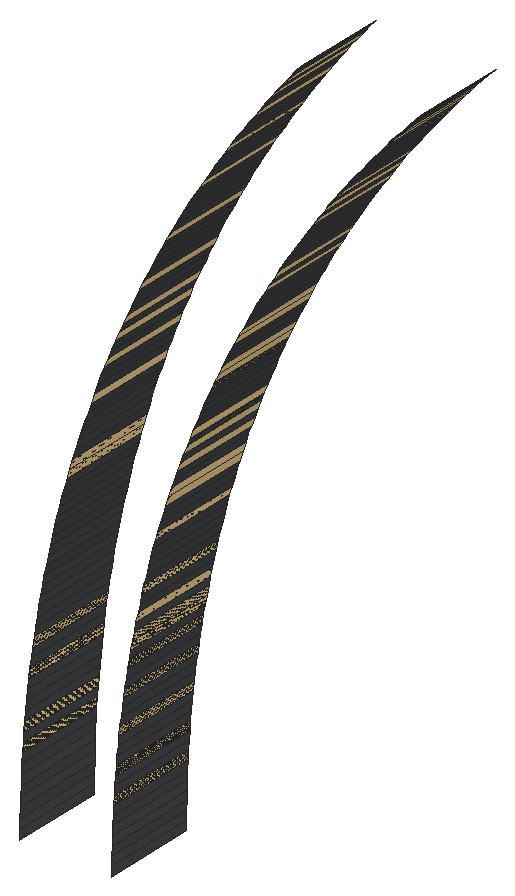
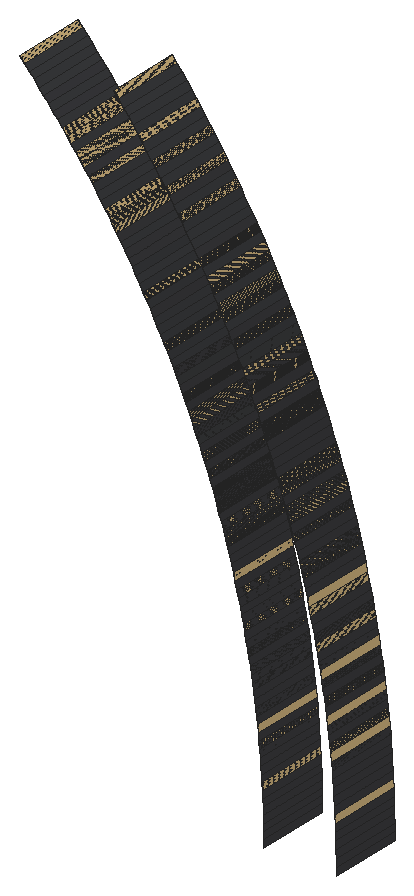
# SketchUp Ruby script. Lengths in inches.
U = 1.inch
M = Sketchup.active_model
def pt(a) = Geom::Point3d.new(a.map { |v| v * U })
def face(e, loops, mat)
  f = e.add_face(loops[0].map { |a| pt(a) })
  loops[1..].each { |l| e.add_face(l.map { |a| pt(a) }).erase! }
  f.material = f.back_material = mat if mat
  f
end
# faces: each face lists its corners as indices into pts; further lists are holes
def faces(e, pts, list, mat = nil) = list.each { |f| face(e, (f[0].is_a?(Array) ? f : [f]).map { |l| l.map { |i| pts[i] } }, mat) }
# xy, xz, yz: faces in a plane at the given z, y or x. An outline is a flat list of corners, or four numbers for a rectangle; further outlines are holes
def ring(l) = l.size == 4 ? [[l[0], l[1]], [l[2], l[1]], [l[2], l[3]], [l[0], l[3]]] : l.each_slice(2).to_a
def flat(e, list, mat, &to3) = list.each { |f| face(e, (f[0].is_a?(Array) ? f : [f]).map { |l| ring(l).map { |u, v| to3.(u, v) } }, mat) }
def xy(e, z, list, mat = nil) = flat(e, list, mat) { |x, y| [x, y, z] }
def xz(e, y, list, mat = nil) = flat(e, list, mat) { |x, z| [x, y, z] }
def yz(e, x, list, mat = nil) = flat(e, list, mat) { |y, z| [x, y, z] }
def lines(e, pts, list) = list.each { |a, b| e.add_line(pt(pts[a]), pt(pts[b])) }
# prism: a flat outline (further loops are holes) pulled along v
def prism(e, loops, v, mat = nil)
  f = face(e, loops, mat); d = Geom::Vector3d.new(v.map { |x| x * U })
  f.pushpull(f.normal.samedirection?(d) ? d.length : -d.length)
end
def box(e, o, s, mat = nil) = prism(e, [[o, [o[0] + s[0], o[1], o[2]], [o[0] + s[0], o[1] + s[1], o[2]], [o[0], o[1] + s[1], o[2]]]], [0, 0, s[2]], mat)
def at(x, y, z, deg = 0) = Geom::Transformation.translation(pt([x, y, z])) * Geom::Transformation.rotation(ORIGIN, Z_AXIS, deg.degrees)
def axes(o, x, y, z) = Geom::Transformation.new([*x, 0, *y, 0, *z, 0, *pt(o).to_a, 1])
def part(name) = M.definitions.add(name)
# library, detail: a bought-in or finely detailed component or shape, given as its bounding box
def library(name, o, s) = part(name).tap { |d| box(d.entities, o, s) }
def detail(e, o, s) = box(e.add_group.entities, o, s)
def put(e, d, t, mat = nil) = e.add_instance(d, t).tap { |i| i.material = mat if mat }
def group(e, t, mat = nil) = e.add_group.tap { |g| g.transformation = t; g.material = mat if mat }.entities
root = M.entities
M.materials.add("1432 AP 8245 TAR ROAD").color = [71, 72, 75]
M.materials.add("Outer Light").color = [251, 217, 152]
yz(root,258.5,[[95.37,560.79,96.87,560.95],[95.37,560.95,96.87,561.11]],"1432 AP 8245 TAR ROAD")
yz(root,258.5,[[95.37,560.79,96.87,560.95],[95.37,560.95,96.87,561.11]],"Outer Light")
yz(root,258.51,[[95.37,561.28,96.87,561.4375]],"1432 AP 8245 TAR ROAD")
yz(root,258.51,[[95.37,561.28,96.87,561.4375]],"Outer Light")
yz(root,258.52,[[95.37,561.6,96.87,561.76]],"1432 AP 8245 TAR ROAD")
yz(root,258.52,[[95.37,561.6,96.87,561.76]],"Outer Light")
yz(root,260,[[95.37,560.79,96.87,560.94],[95.37,560.94,96.87,561.09]],"1432 AP 8245 TAR ROAD")
yz(root,260,[[95.37,560.79,96.87,560.94],[95.37,560.94,96.87,561.09]],"Outer Light")
yz(root,260.01,[[95.37,561.24,96.87,561.39],[95.37,561.39,96.87,561.54]],"1432 AP 8245 TAR ROAD")
yz(root,260.01,[[95.37,561.24,96.87,561.39],[95.37,561.39,96.87,561.54]],"Outer Light")
p = [[258.51,95.37,561.28],[258.5,95.37,561.11],[258.5,96.87,561.11],[258.51,96.87,561.28],[258.51,96.87,561.28],[258.5,96.87,561.11],
  [258.5,95.37,561.11],[258.51,95.37,561.28],[260,95.37,561.09],[260.01,95.37,561.24],[260.01,96.87,561.24],[260,96.87,561.09],
  [260,96.87,561.09],[260.01,96.87,561.24],[260.01,95.37,561.24],[260,95.37,561.09],[258.52,95.37,561.6],[258.51,95.37,561.4375],
  [258.51,96.87,561.4375],[258.52,96.87,561.6],[258.52,96.87,561.6],[258.51,96.87,561.4375],[258.51,95.37,561.4375],[258.52,95.37,561.6],
  [260.01,95.37,561.54],[260.02,95.37,561.6875],[260.02,96.87,561.6875],[260.01,96.87,561.54],[260.01,96.87,561.54],[260.02,96.87,561.6875],
  [260.02,95.37,561.6875],[260.01,95.37,561.54],[260.03,95.37,561.84],[260.03,96.87,561.84],[260.03,96.87,561.84],[260.03,95.37,561.84],
  [258.53,95.37,561.92],[258.52,95.37,561.76],[258.52,96.87,561.76],[258.53,96.87,561.92],[258.53,96.87,561.92],[258.52,96.87,561.76],
  [258.52,95.37,561.76],[258.53,95.37,561.92],[260.04,95.37,561.99],[260.04,96.87,561.99],[260.04,96.87,561.99],[260.04,95.37,561.99],
  [258.54,95.37,562.08],[258.54,96.87,562.08],[258.54,96.87,562.08],[258.54,95.37,562.08],[260.05,95.37,562.13],[260.05,96.87,562.13],
  [260.05,96.87,562.13],[260.05,95.37,562.13],[258.55,95.37,562.24],[258.55,96.87,562.24],[258.55,96.87,562.24],[258.55,95.37,562.24],
  [260.06,95.37,562.28],[260.06,96.87,562.28],[260.06,96.87,562.28],[260.06,95.37,562.28],[258.5625,95.37,562.4],[258.5625,96.87,562.4],
  [258.5625,96.87,562.4],[258.5625,95.37,562.4],[260.07,95.37,562.43],[260.07,96.87,562.43],[260.07,96.87,562.43],[260.07,95.37,562.43],
  [258.58,95.37,562.5625],[258.58,96.87,562.5625],[258.58,96.87,562.5625],[258.58,95.37,562.5625],[260.08,95.37,562.58],[260.08,96.87,562.58],
  [260.08,96.87,562.58],[260.08,95.37,562.58],[258.59,95.37,562.72],[258.59,96.87,562.72],[258.59,96.87,562.72],[258.59,95.37,562.72],
  [260.1,95.37,562.73],[260.1,96.87,562.73],[260.1,96.87,562.73],[260.1,95.37,562.73],[258.61,95.37,562.88],[258.61,96.87,562.88],
  [258.61,96.87,562.88],[258.61,95.37,562.88],[260.11,95.37,562.88],[260.11,96.87,562.88],[260.11,96.87,562.88],[260.11,95.37,562.88],
  [258.625,95.37,563.04],[258.625,96.87,563.04],[258.625,96.87,563.04],[258.625,95.37,563.04],[260.13,95.37,563.03],[260.13,96.87,563.03],
  [260.13,96.87,563.03],[260.13,95.37,563.03],[258.64,95.37,563.2],[258.64,96.87,563.2],[258.64,96.87,563.2],[258.64,95.37,563.2],
  [260.15,95.37,563.17],[260.15,96.87,563.17],[260.15,96.87,563.17],[260.15,95.37,563.17],[258.66,95.37,563.36],[258.66,96.87,563.36],
  [258.66,96.87,563.36],[258.66,95.37,563.36],[260.17,95.37,563.32],[260.17,96.87,563.32],[260.17,96.87,563.32],[260.17,95.37,563.32],
  [260.19,95.37,563.47],[260.19,96.87,563.47],[260.19,96.87,563.47],[260.19,95.37,563.47],[258.68,95.37,563.52],[258.68,96.87,563.52],
  [258.68,96.87,563.52],[258.68,95.37,563.52],[258.7,95.37,563.68],[258.7,96.87,563.68],[258.7,96.87,563.68],[258.7,95.37,563.68],
  [260.21,95.37,563.62],[260.21,96.87,563.62],[260.21,96.87,563.62],[260.21,95.37,563.62],[260.23,95.37,563.76],[260.23,96.87,563.76],
  [260.23,96.87,563.76],[260.23,95.37,563.76],[258.73,95.37,563.84],[258.73,96.87,563.84],[258.73,96.87,563.84],[258.73,95.37,563.84],
  [258.75,95.37,564],[258.75,96.87,564],[258.75,96.87,564],[258.75,95.37,564],[260.26,95.37,563.91],[260.26,96.87,563.91],
  [260.26,96.87,563.91],[260.26,95.37,563.91],[260.28,95.37,564.06],[260.28,96.87,564.06],[260.28,96.87,564.06],[260.28,95.37,564.06],
  [258.78,95.37,564.16],[258.78,96.87,564.16],[258.78,96.87,564.16],[258.78,95.37,564.16],[260.31,95.37,564.21],[260.31,96.87,564.21],
  [260.31,96.87,564.21],[260.31,95.37,564.21],[258.81,95.37,564.32],[258.81,96.87,564.32],[258.81,96.87,564.32],[258.81,95.37,564.32],
  [260.34,95.37,564.35],[260.34,96.87,564.35],[260.34,96.87,564.35],[260.34,95.37,564.35],[258.83,95.37,564.48],[258.83,96.87,564.48],
  [258.83,96.87,564.48],[258.83,95.37,564.48],[260.37,95.37,564.5],[260.37,96.87,564.5],[260.37,96.87,564.5],[260.37,95.37,564.5],
  [258.86,95.37,564.63],[258.86,96.87,564.63],[258.86,96.87,564.63],[258.86,95.37,564.63],[260.39,95.37,564.65],[260.39,96.87,564.65],
  [260.39,96.87,564.65],[260.39,95.37,564.65],[258.89,95.37,564.79],[258.89,96.87,564.79],[258.89,96.87,564.79],[258.89,95.37,564.79],
  [260.43,95.37,564.79],[260.43,96.87,564.79],[260.43,96.87,564.79],[260.43,95.37,564.79],[258.93,95.37,564.95],[258.93,96.87,564.95],
  [258.93,96.87,564.95],[258.93,95.37,564.95],[260.46,95.37,564.9375],[260.46,96.87,564.9375],[260.46,96.87,564.9375],[260.46,95.37,564.9375],
  [258.96,95.37,565.11],[258.96,96.87,565.11],[258.96,96.87,565.11],[258.96,95.37,565.11],[260.49,95.37,565.08],[260.49,96.87,565.08],
  [260.49,96.87,565.08],[260.49,95.37,565.08],[258.99,95.37,565.26],[258.99,96.87,565.26],[258.99,96.87,565.26],[258.99,95.37,565.26],
  [260.52,95.37,565.23],[260.52,96.87,565.23],[260.52,96.87,565.23],[260.52,95.37,565.23],[260.56,95.37,565.37],[260.56,96.87,565.37],
  [260.56,96.87,565.37],[260.56,95.37,565.37],[259.03,95.37,565.42],[259.03,96.87,565.42],[259.03,96.87,565.42],[259.03,95.37,565.42],
  [259.07,95.37,565.58],[259.07,96.87,565.58],[259.07,96.87,565.58],[259.07,95.37,565.58],[260.6,95.37,565.52],[260.6,96.87,565.52],
  [260.6,96.87,565.52],[260.6,95.37,565.52],[260.63,95.37,565.66],[260.63,96.87,565.66],[260.63,96.87,565.66],[260.63,95.37,565.66],
  [259.1,95.37,565.73],[259.1,96.87,565.73],[259.1,96.87,565.73],[259.1,95.37,565.73],[259.14,95.37,565.89],[259.14,96.87,565.89],
  [259.14,96.87,565.89],[259.14,95.37,565.89],[260.67,95.37,565.81],[260.67,96.87,565.81],[260.67,96.87,565.81],[260.67,95.37,565.81],
  [260.71,95.37,565.95],[260.71,96.87,565.95],[260.71,96.87,565.95],[260.71,95.37,565.95],[259.18,95.37,566.05],[259.18,96.87,566.05],
  [259.18,96.87,566.05],[259.18,95.37,566.05],[260.75,95.37,566.09],[260.75,96.87,566.09],[260.75,96.87,566.09],[260.75,95.37,566.09],
  [259.23,95.37,566.2],[259.23,96.87,566.2],[259.23,96.87,566.2],[259.23,95.37,566.2],[260.8,95.37,566.24],[260.8,96.87,566.24],
  [260.8,96.87,566.24],[260.8,95.37,566.24],[259.27,95.37,566.36],[259.27,96.87,566.36],[259.27,96.87,566.36],[259.27,95.37,566.36],
  [260.84,95.37,566.38],[260.84,96.87,566.38],[260.84,96.87,566.38],[260.84,95.37,566.38],[259.3125,95.37,566.51],[259.3125,96.87,566.51],
  [259.3125,96.87,566.51],[259.3125,95.37,566.51],[260.88,95.37,566.52],[260.88,96.87,566.52],[260.88,96.87,566.52],[260.88,95.37,566.52],
  [259.36,95.37,566.67],[259.36,96.87,566.67],[259.36,96.87,566.67],[259.36,95.37,566.67],[260.93,95.37,566.66],[260.93,96.87,566.66],
  [260.93,96.87,566.66],[260.93,95.37,566.66],[259.41,95.37,566.82],[259.41,96.87,566.82],[259.41,96.87,566.82],[259.41,95.37,566.82],
  [260.98,95.37,566.81],[260.98,96.87,566.81],[260.98,96.87,566.81],[260.98,95.37,566.81],[259.45,95.37,566.97],[259.45,96.87,566.97],
  [259.45,96.87,566.97],[259.45,95.37,566.97],[261.02,95.37,566.95],[261.02,96.87,566.95],[261.02,96.87,566.95],[261.02,95.37,566.95],
  [261.07,95.37,567.09],[261.07,96.87,567.09],[261.07,96.87,567.09],[261.07,95.37,567.09],[259.5,95.37,567.125],[259.5,96.87,567.125],
  [259.5,96.87,567.125],[259.5,95.37,567.125],[259.55,95.37,567.28],[259.55,96.87,567.28],[259.55,96.87,567.28],[259.55,95.37,567.28],
  [261.125,95.37,567.23],[261.125,96.87,567.23],[261.125,96.87,567.23],[261.125,95.37,567.23],[261.17,95.37,567.37],[261.17,96.87,567.37],
  [261.17,96.87,567.37],[261.17,95.37,567.37],[259.61,95.37,567.43],[259.61,96.87,567.43],[259.61,96.87,567.43],[259.61,95.37,567.43],
  [259.66,95.37,567.58],[259.66,96.87,567.58],[259.66,96.87,567.58],[259.66,95.37,567.58],[261.23,95.37,567.51],[261.23,96.87,567.51],
  [261.23,96.87,567.51],[261.23,95.37,567.51],[261.28,95.37,567.65],[261.28,96.87,567.65],[261.28,96.87,567.65],[261.28,95.37,567.65],
  [259.71,95.37,567.74],[259.71,96.87,567.74],[259.71,96.87,567.74],[259.71,95.37,567.74],[261.33,95.37,567.79],[261.33,96.87,567.79],
  [261.33,96.87,567.79],[261.33,95.37,567.79],[259.77,95.37,567.89],[259.77,96.87,567.89],[259.77,96.87,567.89],[259.77,95.37,567.89],
  [261.39,95.37,567.92],[261.39,96.87,567.92],[261.39,96.87,567.92],[261.39,95.37,567.92],[259.82,95.37,568.04],[259.82,96.87,568.04],
  [259.82,96.87,568.04],[259.82,95.37,568.04],[261.45,95.37,568.0625],[261.45,96.87,568.0625],[261.45,96.87,568.0625],[261.45,95.37,568.0625],
  [259.88,95.37,568.1875],[259.88,96.87,568.1875],[259.88,96.87,568.1875],[259.88,95.37,568.1875],[261.5,95.37,568.2],[261.5,96.87,568.2],
  [261.5,96.87,568.2],[261.5,95.37,568.2],[259.94,95.37,568.34],[259.94,96.87,568.34],[259.94,96.87,568.34],[259.94,95.37,568.34],
  [261.5625,95.37,568.34],[261.5625,96.87,568.34],[261.5625,96.87,568.34],[261.5625,95.37,568.34],[260,95.37,568.49],[260,96.87,568.49],
  [260,96.87,568.49],[260,95.37,568.49],[261.62,95.37,568.47],[261.62,96.87,568.47],[261.62,96.87,568.47],[261.62,95.37,568.47],
  [260.06,95.37,568.64],[260.06,96.87,568.64],[260.06,96.87,568.64],[260.06,95.37,568.64],[261.68,95.37,568.61],[261.68,96.87,568.61],
  [261.68,96.87,568.61],[261.68,95.37,568.61],[260.12,95.37,568.79],[260.12,96.87,568.79],[260.12,96.87,568.79],[260.12,95.37,568.79],
  [261.75,95.37,568.75],[261.75,96.87,568.75],[261.75,96.87,568.75],[261.75,95.37,568.75],[261.81,95.37,568.88],[261.81,96.87,568.88],
  [261.81,96.87,568.88],[261.81,95.37,568.88],[260.1875,95.37,568.93],[260.1875,96.87,568.93],[260.1875,96.87,568.93],[260.1875,95.37,568.93],
  [260.25,95.37,569.08],[260.25,96.87,569.08],[260.25,96.87,569.08],[260.25,95.37,569.08],[261.87,95.37,569.02],[261.87,96.87,569.02],
  [261.87,96.87,569.02],[261.87,95.37,569.02],[261.9375,95.37,569.15],[261.9375,96.87,569.15],[261.9375,96.87,569.15],[261.9375,95.37,569.15],
  [260.32,95.37,569.23],[260.32,96.87,569.23],[260.32,96.87,569.23],[260.32,95.37,569.23],[260.38,95.37,569.375],[260.38,96.87,569.375],
  [260.38,96.87,569.375],[260.38,95.37,569.375],[262,95.37,569.28],[262,96.87,569.28],[262,96.87,569.28],[262,95.37,569.28],
  [262.07,95.37,569.42],[262.07,96.87,569.42],[262.07,96.87,569.42],[262.07,95.37,569.42],[260.45,95.37,569.52],[260.45,96.87,569.52],
  [260.45,96.87,569.52],[260.45,95.37,569.52],[262.14,95.37,569.55],[262.14,96.87,569.55],[262.14,96.87,569.55],[262.14,95.37,569.55],
  [260.52,95.37,569.67],[260.52,96.87,569.67],[260.52,96.87,569.67],[260.52,95.37,569.67],[262.21,95.37,569.68],[262.21,96.87,569.68],
  [262.21,96.87,569.68],[262.21,95.37,569.68],[260.59,95.37,569.8125],[260.59,96.87,569.8125],[260.59,96.87,569.8125],[260.59,95.37,569.8125],
  [262.28,95.37,569.8125],[262.28,96.87,569.8125],[262.28,96.87,569.8125],[262.28,95.37,569.8125],[260.66,95.37,569.96],[260.66,96.87,569.96],
  [260.66,96.87,569.96],[260.66,95.37,569.96],[262.35,95.37,569.95],[262.35,96.87,569.95],[262.35,96.87,569.95],[262.35,95.37,569.95],
  [262.42,95.37,570.08],[262.42,96.87,570.08],[262.42,96.87,570.08],[262.42,95.37,570.08],[260.73,95.37,570.1],[260.73,96.87,570.1],
  [260.73,96.87,570.1],[260.73,95.37,570.1],[260.81,95.37,570.24],[260.81,96.87,570.24],[260.81,96.87,570.24],[260.81,95.37,570.24],
  [262.5,95.37,570.21],[262.5,96.87,570.21],[262.5,96.87,570.21],[262.5,95.37,570.21],[260.88,95.37,570.38],[260.88,96.87,570.38],
  [260.88,96.87,570.38],[260.88,95.37,570.38],[262.57,95.37,570.34],[262.57,96.87,570.34],[262.57,96.87,570.34],[262.57,95.37,570.34],
  [262.65,95.37,570.46],[262.65,96.87,570.46],[262.65,96.87,570.46],[262.65,95.37,570.46],[260.96,95.37,570.53],[260.96,96.87,570.53],
  [260.96,96.87,570.53],[260.96,95.37,570.53],[261.04,95.37,570.67],[261.04,96.87,570.67],[261.04,96.87,570.67],[261.04,95.37,570.67],
  [262.72,95.37,570.59],[262.72,96.87,570.59],[262.72,96.87,570.59],[262.72,95.37,570.59],[262.8,95.37,570.72],[262.8,96.87,570.72],
  [262.8,96.87,570.72],[262.8,95.37,570.72],[261.11,95.37,570.81],[261.11,96.87,570.81],[261.11,96.87,570.81],[261.11,95.37,570.81],
  [262.88,95.37,570.85],[262.88,96.87,570.85],[262.88,96.87,570.85],[262.88,95.37,570.85],[261.19,95.37,570.95],[261.19,96.87,570.95],
  [261.19,96.87,570.95],[261.19,95.37,570.95],[262.96,95.37,570.97],[262.96,96.87,570.97],[262.96,96.87,570.97],[262.96,95.37,570.97],
  [261.27,95.37,571.09],[261.27,96.87,571.09],[261.27,96.87,571.09],[261.27,95.37,571.09],[263.04,95.37,571.1],[263.04,96.87,571.1],
  [263.04,96.87,571.1],[263.04,95.37,571.1],[261.35,95.37,571.23],[261.35,96.87,571.23],[261.35,96.87,571.23],[261.35,95.37,571.23],
  [263.12,95.37,571.22],[263.12,96.87,571.22],[263.12,96.87,571.22],[263.12,95.37,571.22],[261.4375,95.37,571.37],[261.4375,96.87,571.37],
  [261.4375,96.87,571.37],[261.4375,95.37,571.37],[263.2,95.37,571.35],[263.2,96.87,571.35],[263.2,96.87,571.35],[263.2,95.37,571.35],
  [263.29,95.37,571.47],[263.29,96.87,571.47],[263.29,96.87,571.47],[263.29,95.37,571.47],[261.52,95.37,571.5],[261.52,96.87,571.5],
  [261.52,96.87,571.5],[261.52,95.37,571.5],[261.61,95.37,571.64],[261.61,96.87,571.64],[261.61,96.87,571.64],[261.61,95.37,571.64],
  [263.37,95.37,571.59],[263.37,96.87,571.59],[263.37,96.87,571.59],[263.37,95.37,571.59],[261.69,95.37,571.78],[261.69,96.87,571.78],
  [261.69,96.87,571.78],[261.69,95.37,571.78],[263.46,95.37,571.72],[263.46,96.87,571.72],[263.46,96.87,571.72],[263.46,95.37,571.72],
  [263.54,95.37,571.84],[263.54,96.87,571.84],[263.54,96.87,571.84],[263.54,95.37,571.84],[261.78,95.37,571.91],[261.78,96.87,571.91],
  [261.78,96.87,571.91],[261.78,95.37,571.91],[263.63,95.37,571.96],[263.63,96.87,571.96],[263.63,96.87,571.96],[263.63,95.37,571.96],
  [261.87,95.37,572.05],[261.87,96.87,572.05],[261.87,96.87,572.05],[261.87,95.37,572.05],[261.95,95.37,572.18],[261.95,96.87,572.18],
  [261.95,96.87,572.18],[261.95,95.37,572.18],[263.72,95.37,572.08],[263.72,96.87,572.08],[263.72,96.87,572.08],[263.72,95.37,572.08],
  [263.81,95.37,572.2],[263.81,96.87,572.2],[263.81,96.87,572.2],[263.81,95.37,572.2],[262.04,95.37,572.31],[262.04,96.87,572.31],
  [262.04,96.87,572.31],[262.04,95.37,572.31],[263.9,95.37,572.32],[263.9,96.87,572.32],[263.9,96.87,572.32],[263.9,95.37,572.32],
  [262.14,95.37,572.45],[262.14,96.87,572.45],[262.14,96.87,572.45],[262.14,95.37,572.45],[263.99,95.37,572.4375],[263.99,96.87,572.4375],
  [263.99,96.87,572.4375],[263.99,95.37,572.4375],[262.23,95.37,572.58],[262.23,96.87,572.58],[262.23,96.87,572.58],[262.23,95.37,572.58],
  [264.08,95.37,572.55],[264.08,96.87,572.55],[264.08,96.87,572.55],[264.08,95.37,572.55],[262.32,95.37,572.71],[262.32,96.87,572.71],
  [262.32,96.87,572.71],[262.32,95.37,572.71],[264.17,95.37,572.67],[264.17,96.87,572.67],[264.17,96.87,572.67],[264.17,95.37,572.67],
  [262.42,95.37,572.84],[262.42,96.87,572.84],[262.42,96.87,572.84],[262.42,95.37,572.84],[264.27,95.37,572.79],[264.27,96.87,572.79],
  [264.27,96.87,572.79],[264.27,95.37,572.79],[262.51,95.37,572.97],[262.51,96.87,572.97],[262.51,96.87,572.97],[262.51,95.37,572.97],
  [264.36,95.37,572.9],[264.36,96.87,572.9],[264.36,96.87,572.9],[264.36,95.37,572.9],[264.46,95.37,573.02],[264.46,96.87,573.02],
  [264.46,96.87,573.02],[264.46,95.37,573.02],[262.61,95.37,573.1],[262.61,96.87,573.1],[262.61,96.87,573.1],[262.61,95.37,573.1],
  [264.55,95.37,573.13],[264.55,96.87,573.13],[264.55,96.87,573.13],[264.55,95.37,573.13],[262.7,95.37,573.23],[262.7,96.87,573.23],
  [262.7,96.87,573.23],[262.7,95.37,573.23],[264.65,95.37,573.24],[264.65,96.87,573.24],[264.65,96.87,573.24],[264.65,95.37,573.24],
  [262.8,95.37,573.36],[262.8,96.87,573.36],[262.8,96.87,573.36],[262.8,95.37,573.36],[264.75,95.37,573.36],[264.75,96.87,573.36],
  [264.75,96.87,573.36],[264.75,95.37,573.36],[262.9,95.37,573.48],[262.9,96.87,573.48],[262.9,96.87,573.48],[262.9,95.37,573.48],
  [264.85,95.37,573.47],[264.85,96.87,573.47],[264.85,96.87,573.47],[264.85,95.37,573.47],[263,95.37,573.61],[263,96.87,573.61],
  [263,96.87,573.61],[263,95.37,573.61],[264.95,95.37,573.58],[264.95,96.87,573.58],[264.95,96.87,573.58],[264.95,95.37,573.58],
  [263.1,95.37,573.73],[263.1,96.87,573.73],[263.1,96.87,573.73],[263.1,95.37,573.73],[265.05,95.37,573.6875],[265.05,96.87,573.6875],
  [265.05,96.87,573.6875],[265.05,95.37,573.6875]]
faces(root,p,[[0,1,2,3],[8,9,10,11],[16,17,18,19],[24,25,26,27],[25,32,33,26],[36,37,38,39],[32,44,45,33],[48,36,39,49],
  [44,52,53,45],[56,48,49,57],[52,60,61,53],[64,56,57,65],[60,68,69,61],[72,64,65,73],[68,76,77,69],[80,72,73,81],
  [76,84,85,77],[88,80,81,89],[84,92,93,85],[96,88,89,97],[92,100,101,93],[104,96,97,105],[100,108,109,101],[112,104,105,113],
  [108,116,117,109],[116,120,121,117],[124,112,113,125],[128,124,125,129],[120,132,133,121],[132,136,137,133],[140,128,129,141],[144,140,141,145],
  [136,148,149,137],[148,152,153,149],[156,144,145,157],[152,160,161,153],[164,156,157,165],[160,168,169,161],[172,164,165,173],[168,176,177,169],
  [180,172,173,181],[176,184,185,177],[188,180,181,189],[184,192,193,185],[196,188,189,197],[192,200,201,193],[204,196,197,205],[200,208,209,201],
  [212,204,205,213],[208,216,217,209],[216,220,221,217],[224,212,213,225],[228,224,225,229],[220,232,233,221],[232,236,237,233],[240,228,229,241],
  [244,240,241,245],[236,248,249,237],[248,252,253,249],[256,244,245,257],[252,260,261,253],[264,256,257,265],[260,268,269,261],[272,264,265,273],
  [268,276,277,269],[280,272,273,281],[276,284,285,277],[288,280,281,289],[284,292,293,285],[296,288,289,297],[292,300,301,293],[304,296,297,305],
  [300,308,309,301],[308,312,313,309],[316,304,305,317],[320,316,317,321],[312,324,325,313],[324,328,329,325],[332,320,321,333],[336,332,333,337],
  [328,340,341,329],[340,344,345,341],[348,336,337,349],[344,352,353,345],[356,348,349,357],[352,360,361,353],[364,356,357,365],[360,368,369,361],
  [372,364,365,373],[368,376,377,369],[380,372,373,381],[376,384,385,377],[388,380,381,389],[384,392,393,385],[396,388,389,397],[392,400,401,393],
  [404,396,397,405],[400,408,409,401],[408,412,413,409],[416,404,405,417],[420,416,417,421],[412,424,425,413],[424,428,429,425],[432,420,421,433],
  [436,432,433,437],[428,440,441,429],[440,444,445,441],[448,436,437,449],[444,452,453,445],[456,448,449,457],[452,460,461,453],[464,456,457,465],
  [460,468,469,461],[472,464,465,473],[468,476,477,469],[476,480,481,477],[484,472,473,485],[488,484,485,489],[480,492,493,481],[496,488,489,497],
  [492,500,501,493],[500,504,505,501],[508,496,497,509],[512,508,509,513],[504,516,517,505],[516,520,521,517],[524,512,513,525],[520,528,529,521],
  [532,524,525,533],[528,536,537,529],[540,532,533,541],[536,544,545,537],[548,540,541,549],[544,552,553,545],[556,548,549,557],[552,560,561,553],
  [560,564,565,561],[568,556,557,569],[572,568,569,573],[564,576,577,565],[580,572,573,581],[576,584,585,577],[584,588,589,585],[592,580,581,593],
  [588,596,597,589],[600,592,593,601],[604,600,601,605],[596,608,609,597],[608,612,613,609],[616,604,605,617],[612,620,621,613],[624,616,617,625],
  [620,628,629,621],[632,624,625,633],[628,636,637,629],[640,632,633,641],[636,644,645,637],[648,640,641,649],[644,652,653,645],[656,648,649,657],
  [652,660,661,653],[660,664,665,661],[668,656,657,669],[664,672,673,665],[676,668,669,677],[672,680,681,673],[684,676,677,685],[680,688,689,681],
  [692,684,685,693],[688,696,697,689],[700,692,693,701],[696,704,705,697],[708,700,701,709],[704,712,713,705]],"1432 AP 8245 TAR ROAD")
faces(root,p,[[4,5,6,7],[12,13,14,15],[20,21,22,23],[28,29,30,31],[29,34,35,30],[40,41,42,43],[34,46,47,35],[50,40,43,51],
  [46,54,55,47],[58,50,51,59],[54,62,63,55],[66,58,59,67],[62,70,71,63],[74,66,67,75],[70,78,79,71],[82,74,75,83],
  [78,86,87,79],[90,82,83,91],[86,94,95,87],[98,90,91,99],[94,102,103,95],[106,98,99,107],[102,110,111,103],[114,106,107,115],
  [110,118,119,111],[118,122,123,119],[126,114,115,127],[130,126,127,131],[122,134,135,123],[134,138,139,135],[142,130,131,143],[146,142,143,147],
  [138,150,151,139],[150,154,155,151],[158,146,147,159],[154,162,163,155],[166,158,159,167],[162,170,171,163],[174,166,167,175],[170,178,179,171],
  [182,174,175,183],[178,186,187,179],[190,182,183,191],[186,194,195,187],[198,190,191,199],[194,202,203,195],[206,198,199,207],[202,210,211,203],
  [214,206,207,215],[210,218,219,211],[218,222,223,219],[226,214,215,227],[230,226,227,231],[222,234,235,223],[234,238,239,235],[242,230,231,243],
  [246,242,243,247],[238,250,251,239],[250,254,255,251],[258,246,247,259],[254,262,263,255],[266,258,259,267],[262,270,271,263],[274,266,267,275],
  [270,278,279,271],[282,274,275,283],[278,286,287,279],[290,282,283,291],[286,294,295,287],[298,290,291,299],[294,302,303,295],[306,298,299,307],
  [302,310,311,303],[310,314,315,311],[318,306,307,319],[322,318,319,323],[314,326,327,315],[326,330,331,327],[334,322,323,335],[338,334,335,339],
  [330,342,343,331],[342,346,347,343],[350,338,339,351],[346,354,355,347],[358,350,351,359],[354,362,363,355],[366,358,359,367],[362,370,371,363],
  [374,366,367,375],[370,378,379,371],[382,374,375,383],[378,386,387,379],[390,382,383,391],[386,394,395,387],[398,390,391,399],[394,402,403,395],
  [406,398,399,407],[402,410,411,403],[410,414,415,411],[418,406,407,419],[422,418,419,423],[414,426,427,415],[426,430,431,427],[434,422,423,435],
  [438,434,435,439],[430,442,443,431],[442,446,447,443],[450,438,439,451],[446,454,455,447],[458,450,451,459],[454,462,463,455],[466,458,459,467],
  [462,470,471,463],[474,466,467,475],[470,478,479,471],[478,482,483,479],[486,474,475,487],[490,486,487,491],[482,494,495,483],[498,490,491,499],
  [494,502,503,495],[502,506,507,503],[510,498,499,511],[514,510,511,515],[506,518,519,507],[518,522,523,519],[526,514,515,527],[522,530,531,523],
  [534,526,527,535],[530,538,539,531],[542,534,535,543],[538,546,547,539],[550,542,543,551],[546,554,555,547],[558,550,551,559],[554,562,563,555],
  [562,566,567,563],[570,558,559,571],[574,570,571,575],[566,578,579,567],[582,574,575,583],[578,586,587,579],[586,590,591,587],[594,582,583,595],
  [590,598,599,591],[602,594,595,603],[606,602,603,607],[598,610,611,599],[610,614,615,611],[618,606,607,619],[614,622,623,615],[626,618,619,627],
  [622,630,631,623],[634,626,627,635],[630,638,639,631],[642,634,635,643],[638,646,647,639],[650,642,643,651],[646,654,655,647],[658,650,651,659],
  [654,662,663,655],[662,666,667,663],[670,658,659,671],[666,674,675,667],[678,670,671,679],[674,682,683,675],[686,678,679,687],[682,690,691,683],
  [694,686,687,695],[690,698,699,691],[702,694,695,703],[698,706,707,699],[710,702,703,711],[706,714,715,707]],"Outer Light")
